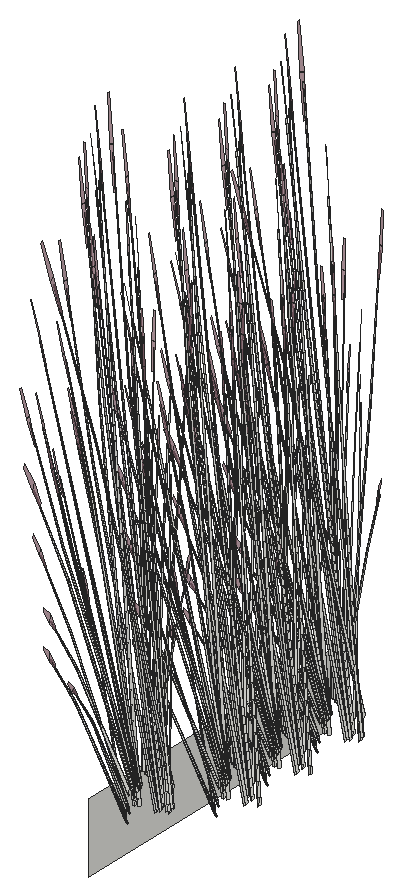
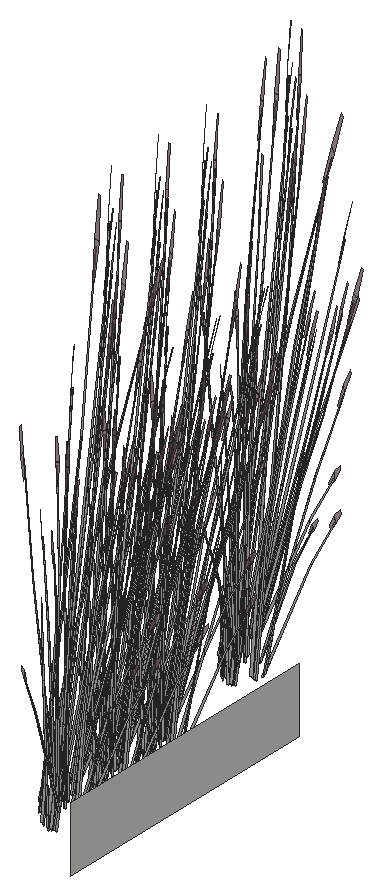
# SketchUp Ruby script. Lengths in inches.
U = 1.inch
M = Sketchup.active_model
def pt(a) = Geom::Point3d.new(a.map { |v| v * U })
def face(e, loops, mat)
  f = e.add_face(loops[0].map { |a| pt(a) })
  loops[1..].each { |l| e.add_face(l.map { |a| pt(a) }).erase! }
  f.material = f.back_material = mat if mat
  f
end
# faces: each face lists its corners as indices into pts; further lists are holes
def faces(e, pts, list, mat = nil) = list.each { |f| face(e, (f[0].is_a?(Array) ? f : [f]).map { |l| l.map { |i| pts[i] } }, mat) }
# xy, xz, yz: faces in a plane at the given z, y or x. An outline is a flat list of corners, or four numbers for a rectangle; further outlines are holes
def ring(l) = l.size == 4 ? [[l[0], l[1]], [l[2], l[1]], [l[2], l[3]], [l[0], l[3]]] : l.each_slice(2).to_a
def flat(e, list, mat, &to3) = list.each { |f| face(e, (f[0].is_a?(Array) ? f : [f]).map { |l| ring(l).map { |u, v| to3.(u, v) } }, mat) }
def xy(e, z, list, mat = nil) = flat(e, list, mat) { |x, y| [x, y, z] }
def xz(e, y, list, mat = nil) = flat(e, list, mat) { |x, z| [x, y, z] }
def yz(e, x, list, mat = nil) = flat(e, list, mat) { |y, z| [x, y, z] }
def lines(e, pts, list) = list.each { |a, b| e.add_line(pt(pts[a]), pt(pts[b])) }
# prism: a flat outline (further loops are holes) pulled along v
def prism(e, loops, v, mat = nil)
  f = face(e, loops, mat); d = Geom::Vector3d.new(v.map { |x| x * U })
  f.pushpull(f.normal.samedirection?(d) ? d.length : -d.length)
end
def box(e, o, s, mat = nil) = prism(e, [[o, [o[0] + s[0], o[1], o[2]], [o[0] + s[0], o[1] + s[1], o[2]], [o[0], o[1] + s[1], o[2]]]], [0, 0, s[2]], mat)
def at(x, y, z, deg = 0) = Geom::Transformation.translation(pt([x, y, z])) * Geom::Transformation.rotation(ORIGIN, Z_AXIS, deg.degrees)
def axes(o, x, y, z) = Geom::Transformation.new([*x, 0, *y, 0, *z, 0, *pt(o).to_a, 1])
def part(name) = M.definitions.add(name)
# library, detail: a bought-in or finely detailed component or shape, given as its bounding box
def library(name, o, s) = part(name).tap { |d| box(d.entities, o, s) }
def detail(e, o, s) = box(e.add_group.entities, o, s)
def put(e, d, t, mat = nil) = e.add_instance(d, t).tap { |i| i.material = mat if mat }
def group(e, t, mat = nil) = e.add_group.tap { |g| g.transformation = t; g.material = mat if mat }.entities
root = M.entities
M.materials.add("LightPink_Translucent").color = [144, 107, 117]
M.materials["LightPink_Translucent"].alpha = 0.75
c1 = part("blade")
p = [[2.15,0.21,22],[0,0.17,0],[0.09,0.45,0],[2.18,0.31,22],[2.29,0.31,22],[0.38,0.45,0],
  [2.48,0.24,33],[2.49,0.24,33],[2.48,0.22,33]]
faces(c1.entities,p,[[0,1,2,3],[4,5,2,3],[6,3,4,7],[8,0,3,6]])
c2 = part("seeds")
p = [[0.3,-0.1,1.38],[-0.01,-0.03,1.59],[-0.01,-0.03,0.03],[0.14,-0.07,-0.07],[0.29,-0.03,3],[0.15,0.01,3.11]]
faces(c2.entities,p,[[0,1,2,3],[1,0,4,5]],"LightPink_Translucent")
c3 = part("blade with seeds")
put(c3.entities,c1,at(0,0,0))
put(c3.entities,c2,axes([2.4,0.25,30.99],[1.5799,-0.05474,1.17369],[-0.12525,1.92788,0.29478],[-0.07173,-0.02425,1.56792]))
yz(root,310,[[14,42,40,48]])
put(root,c3,axes([312.47,31.77,46.18],[-0.12522,-0.35963,0.42415],[0.49122,-0.06241,0.34973],[-0.14477,0.08458,0.87768]))
put(root,c3,axes([312.24,17.43,49.33],[0.12971,0.3568,-0.45151],[-0.49122,0.06241,-0.34973],[-0.14077,0.09583,0.86392]))
put(root,c3,axes([312.48,26.27,46.18],[-0.12522,-0.35963,0.42415],[0.49122,-0.06241,0.34973],[-0.14477,0.08458,0.87768]))
put(root,c3,axes([312.38,15.53,49.375],[0.02542,-0.29714,0.05682],[0.38391,0.00815,0.44729],[-0.14706,-0.03109,0.68204]))
put(root,c3,axes([311.47,18.07,49.36],[-0.01255,0.07733,1.54581],[0.35618,0.269,-0.24447],[-0.09325,0.12721,0.12397]))
put(root,c3,axes([312.85,37.5,45.43],[0.09401,-0.13431,1.51428],[0.3944,0.27795,0.12244],[-0.17792,0.17323,0.64734]))
put(root,c3,axes([312.72,29.99,46.5],[0.41698,-0.28837,0.47505],[0.35962,0.30624,0.3917],[-0.19563,-0.05319,0.983]))
put(root,c3,axes([312.73,24.48,46.5],[0.41698,-0.28837,0.47505],[0.35962,0.30624,0.3917],[-0.19563,-0.05319,0.983]))
put(root,c3,axes([313.46,17.17,47.02],[-0.52523,-0.06406,-0.55095],[0.11084,-0.39517,-0.1446],[-0.15674,-0.04788,1.21613]))
put(root,c3,axes([313.56,15.02,49.99],[-0.33698,0.3746,-0.12034],[-0.48801,-0.21581,-0.66795],[-0.16964,-0.10584,1.01494]))
put(root,c3,axes([312.37,31.71,46.18],[-0.34663,-0.16434,0.05682],[0.20181,-0.23402,0.44729],[-0.11113,0.07566,0.68204]))
put(root,c3,axes([312.38,26.2,46.18],[-0.34663,-0.16434,0.05682],[0.20181,-0.23402,0.44729],[-0.11113,0.07566,0.68204]))
put(root,c3,axes([312.64,15.75,49.66],[0.28729,0.24465,0.31292],[-0.32804,0.23159,-0.40398],[-0.16667,-0.03524,0.77298]))
put(root,c3,axes([312.48,36.5625,46.46],[0.41962,0.10901,0.31292],[-0.12239,0.31802,-0.40398],[-0.16894,0.02916,0.77298]))
put(root,c3,axes([313.41,15.32,49.6],[-0.43054,-0.18887,-0.62776],[0.30598,-0.33097,0.07576],[-0.15599,-0.11277,0.88802]))
put(root,c3,axes([313.21,15.33,49.33],[-0.49824,0.09289,-0.45151],[-0.08716,-0.35177,-0.34973],[-0.13382,-0.10081,0.86392]))
put(root,c3,axes([313.08,31.83,45.43],[0.09401,-0.13431,1.51428],[0.3944,0.27795,0.12244],[-0.17792,0.17323,0.64734]))
put(root,c3,axes([313.09,26.32,45.43],[0.09401,-0.13431,1.51428],[0.3944,0.27795,0.12244],[-0.17792,0.17323,0.64734]))
put(root,c3,axes([312.55,37.55,46.14],[0.12971,0.3568,-0.45151],[-0.49122,0.06241,-0.34973],[-0.14077,0.09583,0.86392]))
put(root,c3,axes([312.6875,35.66,46.18],[0.02542,-0.29714,0.05682],[0.38391,0.00815,0.44729],[-0.14706,-0.03109,0.68204]))
put(root,c3,axes([311.78,38.19,46.17],[-0.01255,0.07733,1.54581],[0.35618,0.269,-0.24447],[-0.09325,0.12721,0.12397]))
put(root,c3,axes([313.78,37.3,43.82],[-0.52523,-0.06406,-0.55095],[0.11084,-0.39517,-0.1446],[-0.15674,-0.04788,1.21613]))
put(root,c3,axes([312.78,17.92,46.98],[-0.47255,-0.19538,-0.43871],[0.28245,-0.35034,0],[-0.10763,-0.0445,1.3917]))
put(root,c3,axes([313.87,35.14,46.8],[-0.33698,0.3746,-0.12034],[-0.48801,-0.21581,-0.66795],[-0.16964,-0.10584,1.01494]))
put(root,c3,axes([312.7,30.89,46.46],[0.41962,0.10901,0.31292],[-0.12239,0.31802,-0.40398],[-0.16894,0.02916,0.77298]))
put(root,c3,axes([312.57,15.01,46.52],[-0.04891,0.05148,1.55816],[-0.49427,0.11098,-0.23804],[-0.1194,-0.10096,0.26541]))
put(root,c3,axes([312.71,25.39,46.46],[0.41962,0.10901,0.31292],[-0.12239,0.31802,-0.40398],[-0.16894,0.02916,0.77298]))
put(root,c3,axes([312.01,17.17,49.64],[0.46706,0.21546,-0.10745],[-0.26908,0.31203,-0.59638],[-0.13196,0.10846,0.90619]))
put(root,c3,axes([312.95,35.875,46.46],[0.28729,0.24465,0.31292],[-0.32804,0.23159,-0.40398],[-0.16667,-0.03524,0.77298]))
put(root,c3,axes([312.77,31.88,46.14],[0.12971,0.3568,-0.45151],[-0.49122,0.06241,-0.34973],[-0.14077,0.09583,0.86392]))
put(root,c3,axes([313.0625,18.16,47.29],[-0.31568,0.39156,0],[-0.52815,-0.21836,-0.456],[-0.12029,-0.04973,1.44655]))
put(root,c3,axes([312.79,26.38,46.14],[0.12971,0.3568,-0.45151],[-0.49122,0.06241,-0.34973],[-0.14077,0.09583,0.86392]))
put(root,c3,axes([313.72,35.45,46.4],[-0.43054,-0.18887,-0.62776],[0.30598,-0.33097,0.07576],[-0.15599,-0.11277,0.88802]))
put(root,c3,axes([313.52,35.45,46.14],[-0.49824,0.09289,-0.45151],[-0.08716,-0.35177,-0.34973],[-0.13382,-0.10081,0.86392]))
put(root,c3,axes([312.91,29.98,46.18],[0.02542,-0.29714,0.05682],[0.38391,0.00815,0.44729],[-0.14706,-0.03109,0.68204]))
put(root,c3,axes([312.01,32.52,46.17],[-0.01255,0.07733,1.54581],[0.35618,0.269,-0.24447],[-0.09325,0.12721,0.12397]))
put(root,c3,axes([312.92,24.48,46.18],[0.02542,-0.29714,0.05682],[0.38391,0.00815,0.44729],[-0.14706,-0.03109,0.68204]))
put(root,c3,axes([312.02,27.02,46.17],[-0.01255,0.07733,1.54581],[0.35618,0.269,-0.24447],[-0.09325,0.12721,0.12397]))
put(root,c3,axes([314,31.625,43.82],[-0.52523,-0.06406,-0.55095],[0.11084,-0.39517,-0.1446],[-0.15674,-0.04788,1.21613]))
put(root,c3,axes([314.09,29.47,46.8],[-0.33698,0.3746,-0.12034],[-0.48801,-0.21581,-0.66795],[-0.16964,-0.10584,1.01494]))
put(root,c3,axes([314.01,26.12,43.82],[-0.52523,-0.06406,-0.55095],[0.11084,-0.39517,-0.1446],[-0.15674,-0.04788,1.21613]))
put(root,c3,axes([314.11,23.97,46.8],[-0.33698,0.3746,-0.12034],[-0.48801,-0.21581,-0.66795],[-0.16964,-0.10584,1.01494]))
put(root,c3,axes([313.17,30.21,46.46],[0.28729,0.24465,0.31292],[-0.32804,0.23159,-0.40398],[-0.16667,-0.03524,0.77298]))
put(root,c3,axes([313.19,24.7,46.46],[0.28729,0.24465,0.31292],[-0.32804,0.23159,-0.40398],[-0.16667,-0.03524,0.77298]))
put(root,c3,axes([313.09,38.04,43.78],[-0.47255,-0.19538,-0.43871],[0.28245,-0.35034,0],[-0.10763,-0.0445,1.3917]))
put(root,c3,axes([311.24,18.11,50.18],[0.44556,0.1043,-0.05733],[-0.13706,0.32103,-0.25992],[-0.07288,0.04874,0.85731]))
put(root,c3,axes([312.88,35.13,43.32],[-0.04891,0.05148,1.55816],[-0.49427,0.11098,-0.23804],[-0.1194,-0.10096,0.26541]))
put(root,c3,axes([312.32,37.3,46.45],[0.46706,0.21546,-0.10745],[-0.26908,0.31203,-0.59638],[-0.13196,0.10846,0.90619]))
put(root,c3,axes([313.95,29.77,46.4],[-0.43054,-0.18887,-0.62776],[0.30598,-0.33097,0.07576],[-0.15599,-0.11277,0.88802]))
put(root,c3,axes([313.96,24.27,46.4],[-0.43054,-0.18887,-0.62776],[0.30598,-0.33097,0.07576],[-0.15599,-0.11277,0.88802]))
put(root,c3,axes([313.74,29.78,46.14],[-0.49824,0.09289,-0.45151],[-0.08716,-0.35177,-0.34973],[-0.13382,-0.10081,0.86392]))
put(root,c3,axes([313.76,24.28,46.14],[-0.49824,0.09289,-0.45151],[-0.08716,-0.35177,-0.34973],[-0.13382,-0.10081,0.86392]))
put(root,c3,axes([312.24,17.2,49.66],[0.43951,-0.05584,0.31292],[0.11606,0.31924,-0.40398],[-0.12595,0.08575,0.77298]))
put(root,c3,axes([313.375,38.28,44.1],[-0.31568,0.39156,0],[-0.52815,-0.21836,-0.456],[-0.12029,-0.04973,1.44655]))
put(root,c3,axes([312.49,18.72,47.49],[0.15933,-0.06164,1.26356],[0.39339,0.18587,-0.27174],[-0.11709,0.16083,0.54024]))
put(root,c3,axes([312.26,15.21,47.08],[-0.14565,0.31907,-0.0344],[-0.44829,-0.09815,-0.15595],[-0.06806,-0.05219,0.51438]))
put(root,c3,axes([313.31,32.37,43.78],[-0.47255,-0.19538,-0.43871],[0.28245,-0.35034,0],[-0.10763,-0.0445,1.3917]))
put(root,c3,axes([313.32,26.87,43.78],[-0.47255,-0.19538,-0.43871],[0.28245,-0.35034,0],[-0.10763,-0.0445,1.3917]))
put(root,c3,axes([313.1,29.46,43.32],[-0.04891,0.05148,1.55816],[-0.49427,0.11098,-0.23804],[-0.1194,-0.10096,0.26541]))
put(root,c3,axes([312.54,31.625,46.45],[0.46706,0.21546,-0.10745],[-0.26908,0.31203,-0.59638],[-0.13196,0.10846,0.90619]))
put(root,c3,axes([313.11,23.96,43.32],[-0.04891,0.05148,1.55816],[-0.49427,0.11098,-0.23804],[-0.1194,-0.10096,0.26541]))
put(root,c3,axes([312.55,26.12,46.45],[0.46706,0.21546,-0.10745],[-0.26908,0.31203,-0.59638],[-0.13196,0.10846,0.90619]))
put(root,c3,axes([313.43,14.125,49.36],[-0.00942,0.04684,1.56736],[-0.46458,0.16998,-0.1481],[-0.13671,-0.08689,0.27737]))
put(root,c3,axes([311.55,38.23,46.99],[0.44556,0.1043,-0.05733],[-0.13706,0.32103,-0.25992],[-0.07288,0.04874,0.85731]))
put(root,c3,axes([313.6,32.61,44.1],[-0.31568,0.39156,0],[-0.52815,-0.21836,-0.456],[-0.12029,-0.04973,1.44655]))
put(root,c3,axes([313.61,27.11,44.1],[-0.31568,0.39156,0],[-0.52815,-0.21836,-0.456],[-0.12029,-0.04973,1.44655]))
put(root,c3,axes([312.93,14.81,47.49],[-0.03058,0.12783,1.26356],[-0.44698,0.10701,-0.27174],[-0.10448,-0.16522,0.54024]))
put(root,c3,axes([312.55,37.33,46.46],[0.43951,-0.05584,0.31292],[0.11606,0.31924,-0.40398],[-0.12595,0.08575,0.77298]))
put(root,c3,axes([313.08,15.14,48.62],[0.11542,0.12546,1.51428],[-0.53333,0.10562,0.12244],[-0.12054,-0.19696,0.64734]))
put(root,c3,axes([314.06,17.23,47.55],[-0.50979,0.25942,-0.25709],[-0.339,-0.36656,-0.44182],[-0.12578,-0.03723,1.41118]))
put(root,c3,axes([312.8,38.85,44.29],[0.15933,-0.06164,1.26356],[0.39339,0.18587,-0.27174],[-0.11709,0.16083,0.54024]))
put(root,c3,axes([312.65,18.05,49.38],[-0.35954,-0.26661,0.42415],[0.38183,-0.22994,0.34973],[-0.06632,0.12508,0.87768]))
put(root,c3,axes([312.57,35.33,43.88],[-0.14565,0.31907,-0.0344],[-0.44829,-0.09815,-0.15595],[-0.06806,-0.05219,0.51438]))
put(root,c3,axes([311.77,32.5625,46.99],[0.44556,0.1043,-0.05733],[-0.13706,0.32103,-0.25992],[-0.07288,0.04874,0.85731]))
put(root,c3,axes([313.26,15.07,49.2],[-0.07798,-0.31474,-0.31292],[0.44579,-0.08311,0.40398],[-0.11974,-0.09019,0.77298]))
put(root,c3,axes([311.78,27.06,46.99],[0.44556,0.1043,-0.05733],[-0.13706,0.32103,-0.25992],[-0.07288,0.04874,0.85731]))
put(root,c3,axes([312.02,16.66,47.29],[-0.63136,0,0],[0,-0.43672,-0.456],[0,-0.09947,1.44655]))
put(root,c3,axes([312.91,17.77,46.99],[-0.11861,-0.34048,-0.27372],[0.47106,-0.09668,0.27372],[-0.09497,-0.03926,1.22797]))
put(root,c3,axes([312.52,18.02,49.375],[-0.41493,-0.01821,0.05682],[0.01138,-0.27493,0.44729],[-0.04342,0.10531,0.68204]))
put(root,c3,axes([312.77,31.65,46.46],[0.43951,-0.05584,0.31292],[0.11606,0.31924,-0.40398],[-0.12595,0.08575,0.77298]))
put(root,c3,axes([313.74,34.25,46.16],[-0.00942,0.04684,1.56736],[-0.46458,0.16998,-0.1481],[-0.13671,-0.08689,0.27737]))
put(root,c3,axes([312.78,26.15,46.46],[0.43951,-0.05584,0.31292],[0.11606,0.31924,-0.40398],[-0.12595,0.08575,0.77298]))
put(root,c3,axes([312.65,18.13,49.2],[-0.34164,0.20573,-0.31292],[-0.3234,-0.23491,0.40398],[-0.04921,0.11936,0.77298]))
put(root,c3,axes([313.02,33.18,44.29],[0.15933,-0.06164,1.26356],[0.39339,0.18587,-0.27174],[-0.11709,0.16083,0.54024]))
put(root,c3,axes([313.24,34.93,44.29],[-0.03058,0.12783,1.26356],[-0.44698,0.10701,-0.27174],[-0.10448,-0.16522,0.54024]))
put(root,c3,axes([313.03,27.67,44.29],[0.15933,-0.06164,1.26356],[0.39339,0.18587,-0.27174],[-0.11709,0.16083,0.54024]))
put(root,c3,axes([312.79,29.66,43.88],[-0.14565,0.31907,-0.0344],[-0.44829,-0.09815,-0.15595],[-0.06806,-0.05219,0.51438]))
put(root,c3,axes([313.39,35.26,45.43],[0.11542,0.12546,1.51428],[-0.53333,0.10562,0.12244],[-0.12054,-0.19696,0.64734]))
put(root,c3,axes([312.81,24.16,43.88],[-0.14565,0.31907,-0.0344],[-0.44829,-0.09815,-0.15595],[-0.06806,-0.05219,0.51438]))
put(root,c3,axes([314.37,37.35,44.36],[-0.50979,0.25942,-0.25709],[-0.339,-0.36656,-0.44182],[-0.12578,-0.03723,1.41118]))
put(root,c3,axes([312.96,38.17,46.18],[-0.35954,-0.26661,0.42415],[0.38183,-0.22994,0.34973],[-0.06632,0.12508,0.87768]))
put(root,c3,axes([314.4,17.51,47.02],[-0.34009,0.2937,-0.55095],[-0.42248,-0.26632,-0.1446],[-0.13628,0.07327,1.21613]))
put(root,c3,axes([313.96,28.58,46.16],[-0.00942,0.04684,1.56736],[-0.46458,0.16998,-0.1481],[-0.13671,-0.08689,0.27737]))
put(root,c3,axes([313.53,15.33,49.66],[0.07798,0.31474,0.31292],[-0.44579,0.08311,-0.40398],[-0.11974,-0.09019,0.77298]))
put(root,c3,axes([313.57,35.2,46],[-0.07798,-0.31474,-0.31292],[0.44579,-0.08311,0.40398],[-0.11974,-0.09019,0.77298]))
put(root,c3,axes([313.98,23.08,46.16],[-0.00942,0.04684,1.56736],[-0.46458,0.16998,-0.1481],[-0.13671,-0.08689,0.27737]))
put(root,c3,axes([311.43,18.86,49.36],[0.05728,-0.02359,1.56736],[0.47345,0.15692,-0.1481],[-0.01113,0.13066,0.27737]))
put(root,c3,axes([312.33,36.79,44.1],[-0.63136,0,0],[0,-0.43672,-0.456],[0,-0.09947,1.44655]))
put(root,c3,axes([313.22,37.9,43.79],[-0.11861,-0.34048,-0.27372],[0.47106,-0.09668,0.27372],[-0.09497,-0.03926,1.22797]))
put(root,c3,axes([313.46,29.26,44.29],[-0.03058,0.12783,1.26356],[-0.44698,0.10701,-0.27174],[-0.10448,-0.16522,0.54024]))
put(root,c3,axes([312.51,16.55,47.26],[-0.46965,0.32852,0.27176],[-0.46994,-0.32506,-0.32244],[-0.0164,-0.09329,1.45692]))
put(root,c3,axes([312.83,38.15,46.18],[-0.41493,-0.01821,0.05682],[0.01138,-0.27493,0.44729],[-0.04342,0.10531,0.68204]))
put(root,c3,axes([313.48,23.76,44.29],[-0.03058,0.12783,1.26356],[-0.44698,0.10701,-0.27174],[-0.10448,-0.16522,0.54024]))
put(root,c3,axes([313.61,29.59,45.43],[0.11542,0.12546,1.51428],[-0.53333,0.10562,0.12244],[-0.12054,-0.19696,0.64734]))
put(root,c3,axes([313.625,24.09,45.43],[0.11542,0.12546,1.51428],[-0.53333,0.10562,0.12244],[-0.12054,-0.19696,0.64734]))
put(root,c3,axes([312.96,38.25,46],[-0.34164,0.20573,-0.31292],[-0.3234,-0.23491,0.40398],[-0.04921,0.11936,0.77298]))
put(root,c3,axes([314.59,31.68,44.36],[-0.50979,0.25942,-0.25709],[-0.339,-0.36656,-0.44182],[-0.12578,-0.03723,1.41118]))
put(root,c3,axes([314.44,17.46,48.13],[0.43633,0.15757,1.33654],[-0.42745,0.33945,0.52853],[-0.19146,-0.20119,1.12046]))
put(root,c3,axes([314.61,26.18,44.36],[-0.50979,0.25942,-0.25709],[-0.339,-0.36656,-0.44182],[-0.12578,-0.03723,1.41118]))
put(root,c3,axes([313.19,32.5,46.18],[-0.35954,-0.26661,0.42415],[0.38183,-0.22994,0.34973],[-0.06632,0.12508,0.87768]))
put(root,c3,axes([313.2,27,46.18],[-0.35954,-0.26661,0.42415],[0.38183,-0.22994,0.34973],[-0.06632,0.12508,0.87768]))
put(root,c3,axes([312.78,14.6,47.64],[0.26338,0.136,1.01491],[-0.38358,0.08175,0.74569],[-0.08207,-0.10452,0.22354]))
put(root,c3,axes([314.63,17.35,47.375],[-0.49304,-0.31451,-0.2226],[0.41487,-0.35316,0.48713],[-0.13277,0.03679,1.48635]))
put(root,c3,axes([313.8,29.52,46],[-0.07798,-0.31474,-0.31292],[0.44579,-0.08311,0.40398],[-0.11974,-0.09019,0.77298]))
put(root,c3,axes([313.74,17.05,47.15],[-0.30332,-0.32798,-0.39531],[0.45944,-0.23096,0.19025],[-0.09816,-0.04058,1.26923]))
put(root,c3,axes([313.81,24.02,46],[-0.07798,-0.31474,-0.31292],[0.44579,-0.08311,0.40398],[-0.11974,-0.09019,0.77298]))
put(root,c3,axes([312.55,31.12,44.1],[-0.63136,0,0],[0,-0.43672,-0.456],[0,-0.09947,1.44655]))
put(root,c3,axes([313.44,32.23,43.79],[-0.11861,-0.34048,-0.27372],[0.47106,-0.09668,0.27372],[-0.09497,-0.03926,1.22797]))
put(root,c3,axes([312.57,25.61,44.1],[-0.63136,0,0],[0,-0.43672,-0.456],[0,-0.09947,1.44655]))
put(root,c3,axes([313.45,26.72,43.79],[-0.11861,-0.34048,-0.27372],[0.47106,-0.09668,0.27372],[-0.09497,-0.03926,1.22797]))
put(root,c3,axes([314.71,37.64,43.82],[-0.34009,0.2937,-0.55095],[-0.42248,-0.26632,-0.1446],[-0.13628,0.07327,1.21613]))
put(root,c3,axes([313.05,32.48,46.18],[-0.41493,-0.01821,0.05682],[0.01138,-0.27493,0.44729],[-0.04342,0.10531,0.68204]))
put(root,c3,axes([313.07,26.97,46.18],[-0.41493,-0.01821,0.05682],[0.01138,-0.27493,0.44729],[-0.04342,0.10531,0.68204]))
put(root,c3,axes([312.88,17.91,49.91],[-0.01314,0.36145,-0.69681],[-0.55324,-0.02428,0.08409],[-0.05838,0.15313,0.9857]))
put(root,c3,axes([313.84,35.45,46.46],[0.07798,0.31474,0.31292],[-0.44579,0.08311,-0.40398],[-0.11974,-0.09019,0.77298]))
put(root,c3,axes([311.74,38.99,46.16],[0.05728,-0.02359,1.56736],[0.47345,0.15692,-0.1481],[-0.01113,0.13066,0.27737]))
put(root,c3,axes([313.18,32.58,46],[-0.34164,0.20573,-0.31292],[-0.3234,-0.23491,0.40398],[-0.04921,0.11936,0.77298]))
put(root,c3,axes([313.2,27.08,46],[-0.34164,0.20573,-0.31292],[-0.3234,-0.23491,0.40398],[-0.04921,0.11936,0.77298]))
put(root,c3,axes([312.82,36.67,44.06],[-0.46965,0.32852,0.27176],[-0.46994,-0.32506,-0.32244],[-0.0164,-0.09329,1.45692]))
put(root,c3,axes([312.87,18.93,47.64],[-0.01307,-0.23234,1.01491],[0.32652,0.16572,0.74569],[-0.06422,0.11074,0.22354]))
put(root,c3,axes([313.33,14.96,49.7],[0.56246,-0.10044,0.47505],[0.09762,0.39398,0.3917],[-0.13228,-0.11611,0.983]))
put(root,c3,axes([314.38,17.28,47.15],[-0.54829,0.02412,-0.39531],[-0.04958,-0.40041,0.19025],[-0.09816,0.04058,1.26923]))
put(root,c3,axes([314.75,37.58,44.9375],[0.43633,0.15757,1.33654],[-0.42745,0.33945,0.52853],[-0.19146,-0.20119,1.12046]))
put(root,c3,axes([314.93,31.97,43.82],[-0.34009,0.2937,-0.55095],[-0.42248,-0.26632,-0.1446],[-0.13628,0.07327,1.21613]))
put(root,c3,axes([314.95,26.46,43.82],[-0.34009,0.2937,-0.55095],[-0.42248,-0.26632,-0.1446],[-0.13628,0.07327,1.21613]))
put(root,c3,axes([313.09,34.72,44.44],[0.26338,0.136,1.01491],[-0.38358,0.08175,0.74569],[-0.08207,-0.10452,0.22354]))
put(root,c3,axes([314.06,29.78,46.46],[0.07798,0.31474,0.31292],[-0.44579,0.08311,-0.40398],[-0.11974,-0.09019,0.77298]))
put(root,c3,axes([314.94,37.47,44.18],[-0.49304,-0.31451,-0.2226],[0.41487,-0.35316,0.48713],[-0.13277,0.03679,1.48635]))
put(root,c3,axes([314.07,24.28,46.46],[0.07798,0.31474,0.31292],[-0.44579,0.08311,-0.40398],[-0.11974,-0.09019,0.77298]))
put(root,c3,axes([314.05,37.17,43.95],[-0.30332,-0.32798,-0.39531],[0.45944,-0.23096,0.19025],[-0.09816,-0.04058,1.26923]))
put(root,c3,axes([313.46,15.04,49.375],[0.22948,-0.24822,0.05682],[0.32679,0.14452,0.44729],[-0.10565,-0.07958,0.68204]))
put(root,c3,axes([311.97,33.3125,46.16],[0.05728,-0.02359,1.56736],[0.47345,0.15692,-0.1481],[-0.01113,0.13066,0.27737]))
put(root,c3,axes([311.98,27.8125,46.16],[0.05728,-0.02359,1.56736],[0.47345,0.15692,-0.1481],[-0.01113,0.13066,0.27737]))
put(root,c3,axes([313.04,31,44.06],[-0.46965,0.32852,0.27176],[-0.46994,-0.32506,-0.32244],[-0.0164,-0.09329,1.45692]))
put(root,c3,axes([313.06,25.5,44.06],[-0.46965,0.32852,0.27176],[-0.46994,-0.32506,-0.32244],[-0.0164,-0.09329,1.45692]))
put(root,c3,axes([313.19,38.04,46.72],[-0.01314,0.36145,-0.69681],[-0.55324,-0.02428,0.08409],[-0.05838,0.15313,0.9857]))
put(root,c3,axes([313.34,17.95,47.39],[0.47255,0.19538,0.43871],[-0.28245,0.35034,0],[-0.10763,-0.0445,1.3917]))
